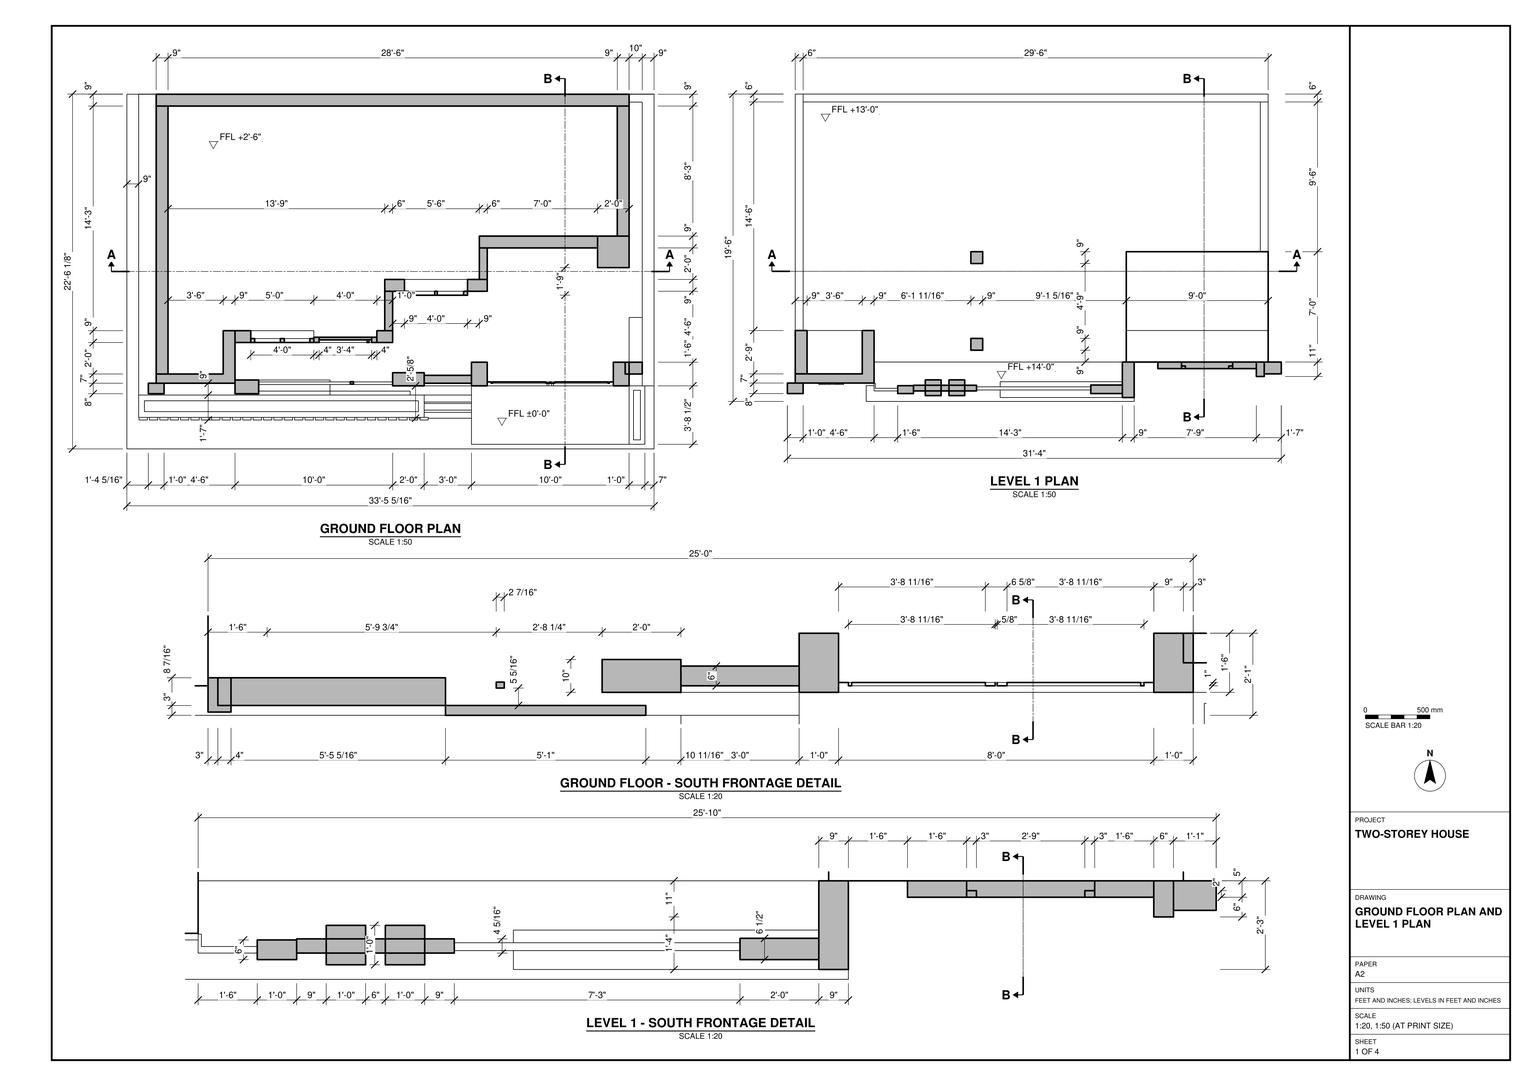
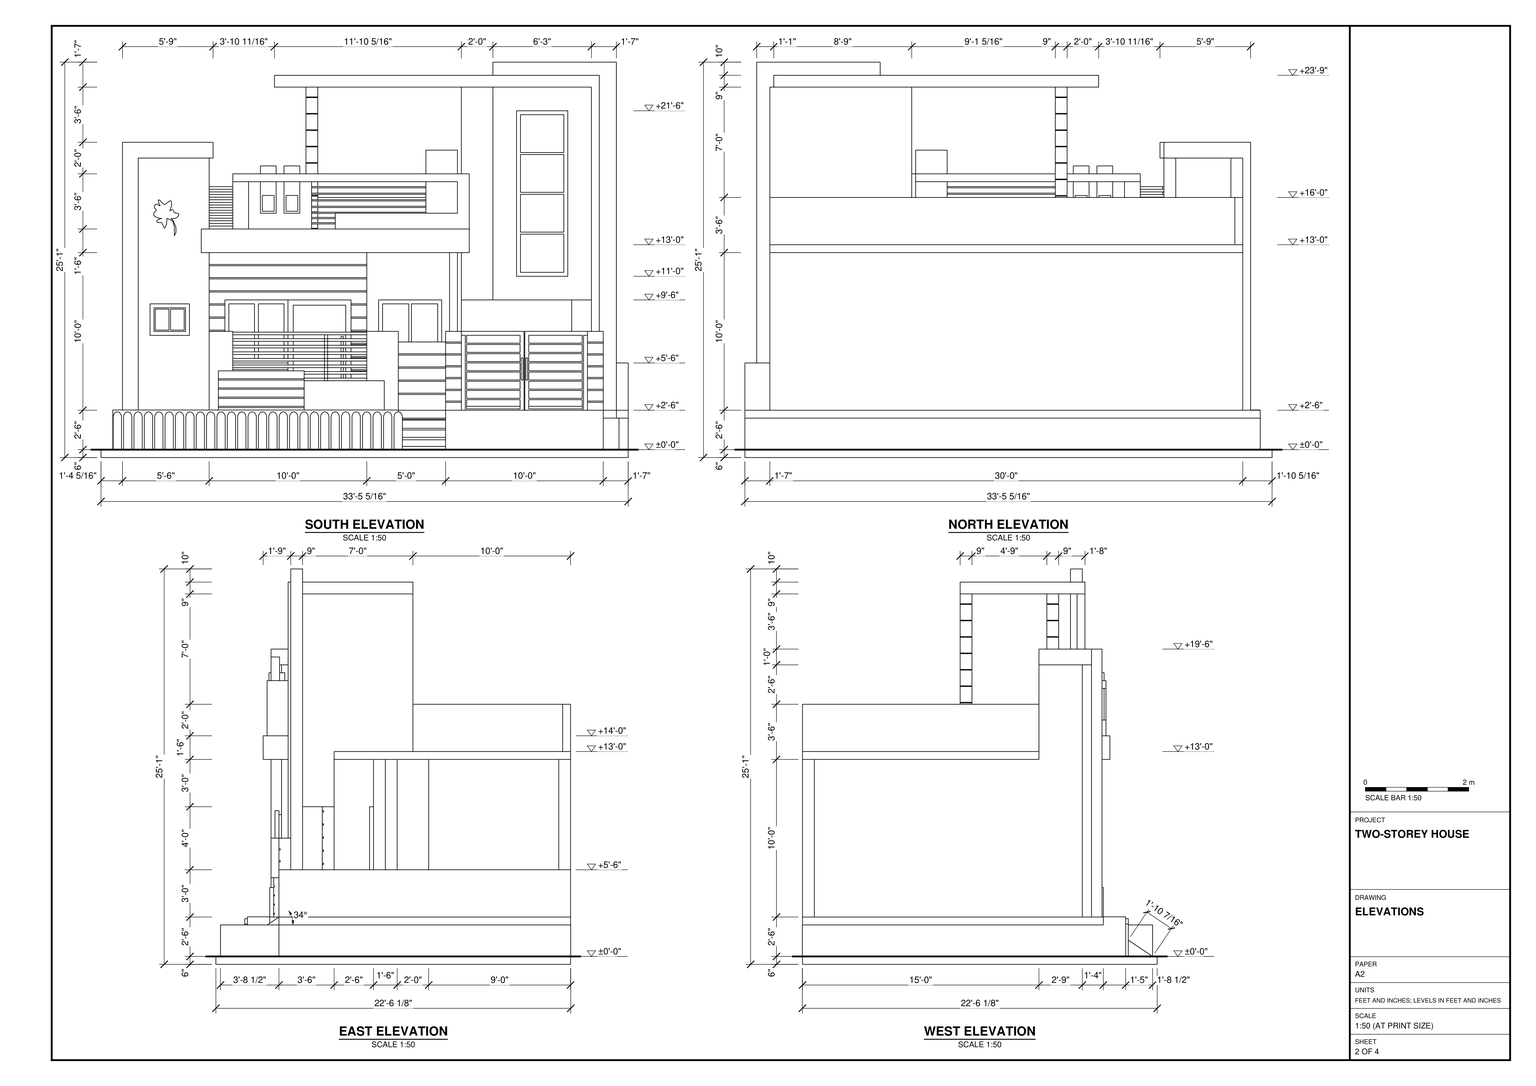
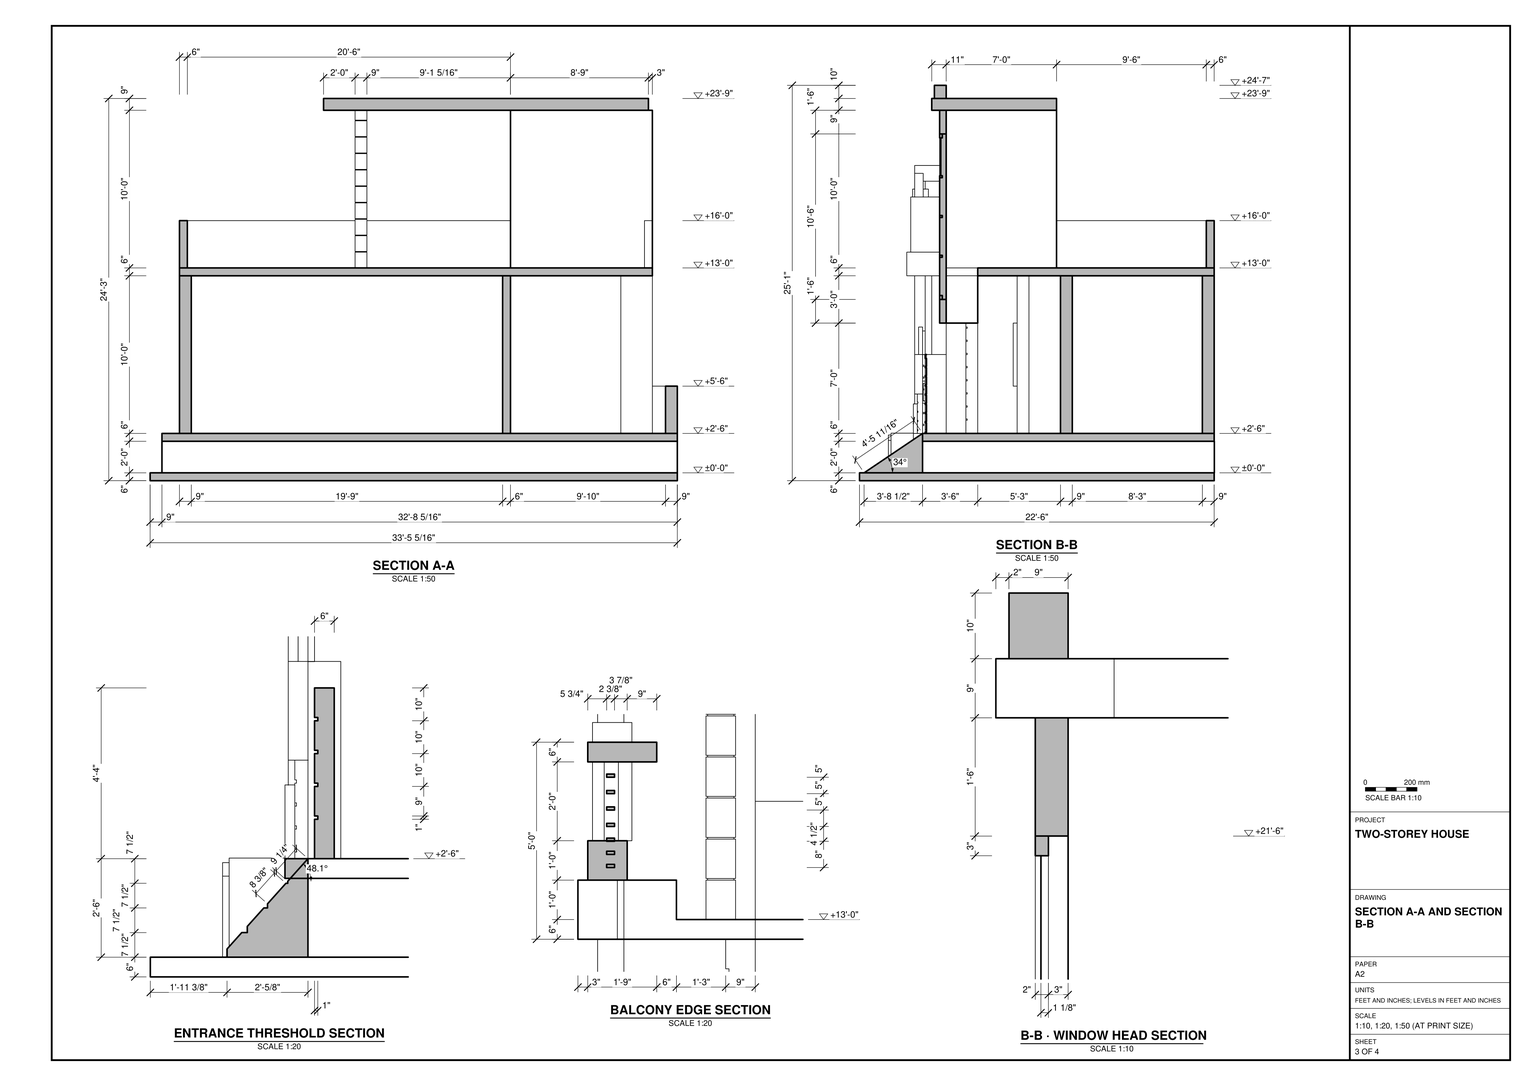
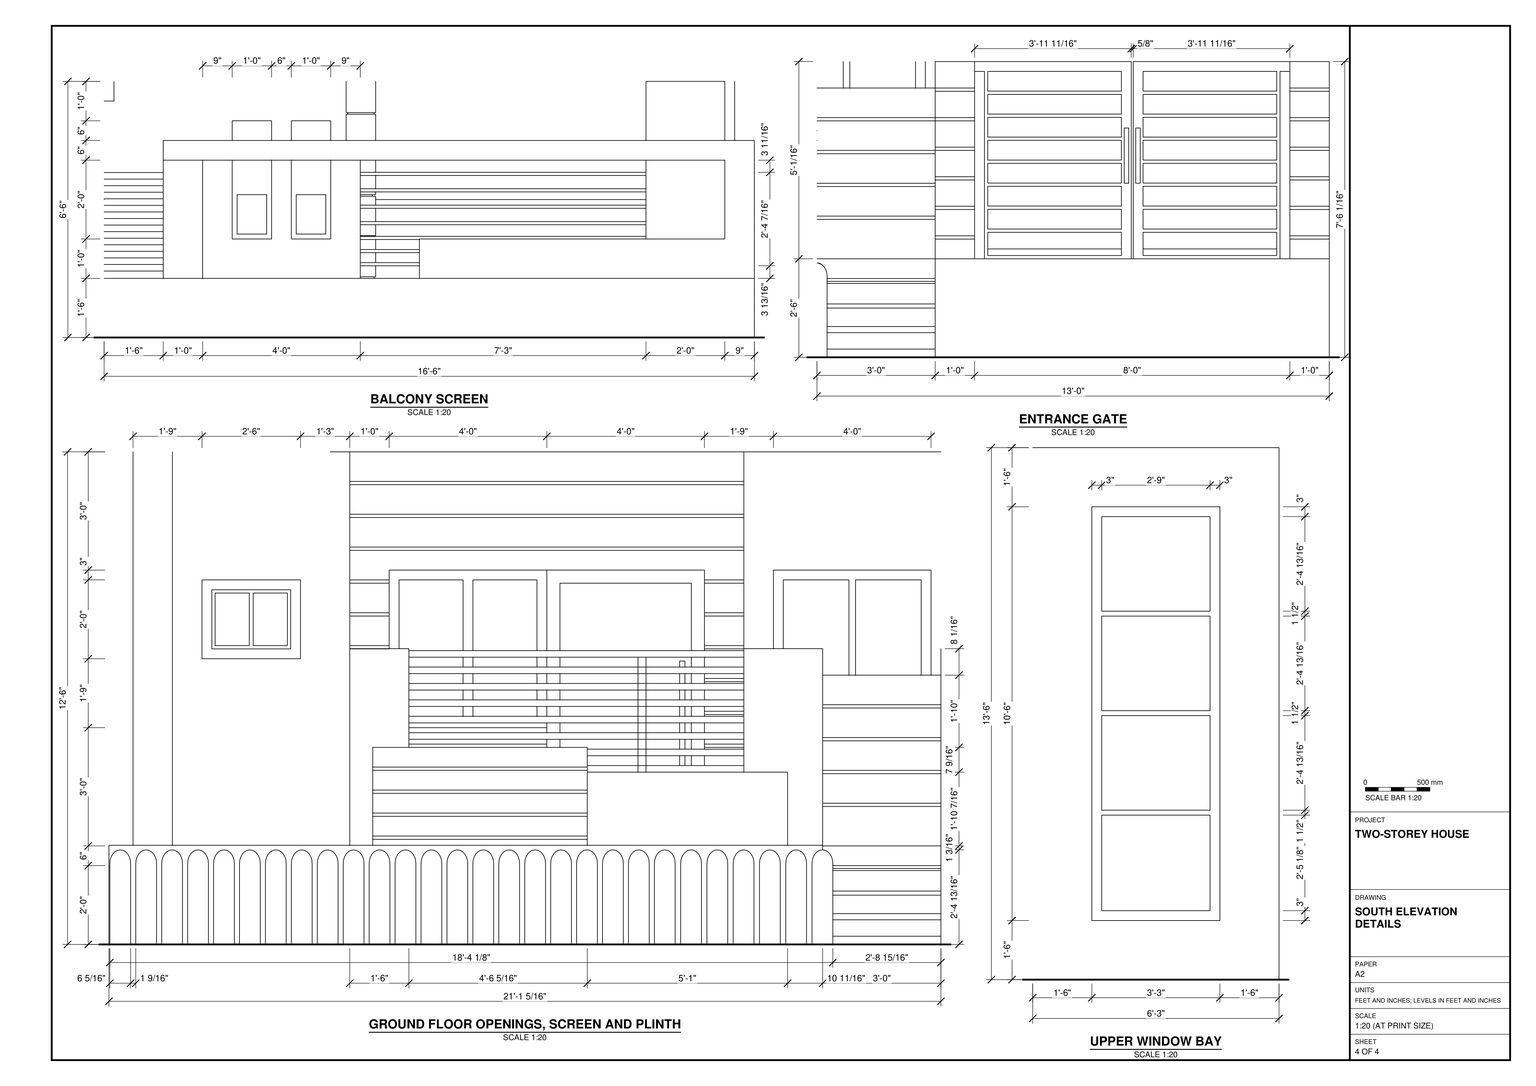
Build the two-storey house in SketchUp using task_files/diagram_01.pdf. Work in feet and inches. The model, including its base, is 33'-5 5/16" wide along X, 22'-6 1/8" deep along Y and 25'-1" high. Use ±0'-0" as the ground datum and +13'-0" as the Level 1 floor level. The raised ground-floor surface is at +2'-6".

Follow the plans for the wall runs, including the stepped outline behind the south frontage. Use the 9" and 6" wall thicknesses where indicated. Use the sections to set the base, plinth, floor slabs, parapets and flat roof canopy. Leave the upper terrace open where the canopy does not cover it.

Build the front approach with the entrance steps and the adjacent ramp leading to the paired gate. Use the enlarged frontage details to position the posts, low walls and horizontal rails. Set the door and window units into the wall openings. On the upper frontage, model the projecting balcony edge, its railing, the canopy supports and the tall window with stacked panes on the right.

Keep walls, slabs and roof elements in separate groups or components. Group each furniture or joinery piece shown separately, and use components for repeated parts. Decor and loose items shown may be any suitable library components. Save one SketchUp model as output_files/two_storey_house_with_a_south_facing_balcony.skp.

# SketchUp Ruby script. Lengths in inches.
U = 1.inch
M = Sketchup.active_model
def pt(a) = Geom::Point3d.new(a.map { |v| v * U })
def face(e, loops, mat)
  f = e.add_face(loops[0].map { |a| pt(a) })
  loops[1..].each { |l| e.add_face(l.map { |a| pt(a) }).erase! }
  f.material = f.back_material = mat if mat
  f
end
# faces: each face lists its corners as indices into pts; further lists are holes
def faces(e, pts, list, mat = nil) = list.each { |f| face(e, (f[0].is_a?(Array) ? f : [f]).map { |l| l.map { |i| pts[i] } }, mat) }
# xy, xz, yz: faces in a plane at the given z, y or x. An outline is a flat list of corners, or four numbers for a rectangle; further outlines are holes
def ring(l) = l.size == 4 ? [[l[0], l[1]], [l[2], l[1]], [l[2], l[3]], [l[0], l[3]]] : l.each_slice(2).to_a
def flat(e, list, mat, &to3) = list.each { |f| face(e, (f[0].is_a?(Array) ? f : [f]).map { |l| ring(l).map { |u, v| to3.(u, v) } }, mat) }
def xy(e, z, list, mat = nil) = flat(e, list, mat) { |x, y| [x, y, z] }
def xz(e, y, list, mat = nil) = flat(e, list, mat) { |x, z| [x, y, z] }
def yz(e, x, list, mat = nil) = flat(e, list, mat) { |y, z| [x, y, z] }
def lines(e, pts, list) = list.each { |a, b| e.add_line(pt(pts[a]), pt(pts[b])) }
# prism: a flat outline (further loops are holes) pulled along v
def prism(e, loops, v, mat = nil)
  f = face(e, loops, mat); d = Geom::Vector3d.new(v.map { |x| x * U })
  f.pushpull(f.normal.samedirection?(d) ? d.length : -d.length)
end
def box(e, o, s, mat = nil) = prism(e, [[o, [o[0] + s[0], o[1], o[2]], [o[0] + s[0], o[1] + s[1], o[2]], [o[0], o[1] + s[1], o[2]]]], [0, 0, s[2]], mat)
def at(x, y, z, deg = 0) = Geom::Transformation.translation(pt([x, y, z])) * Geom::Transformation.rotation(ORIGIN, Z_AXIS, deg.degrees)
def axes(o, x, y, z) = Geom::Transformation.new([*x, 0, *y, 0, *z, 0, *pt(o).to_a, 1])
def part(name) = M.definitions.add(name)
# library, detail: a bought-in or finely detailed component or shape, given as its bounding box
def library(name, o, s) = part(name).tap { |d| box(d.entities, o, s) }
def detail(e, o, s) = box(e.add_group.entities, o, s)
def put(e, d, t, mat = nil) = e.add_instance(d, t).tap { |i| i.material = mat if mat }
def group(e, t, mat = nil) = e.add_group.tap { |g| g.transformation = t; g.material = mat if mat }.entities
root = M.entities
M.materials.add("[Cladding Stucco White]").color = [200, 200, 200]
M.materials.add("[Color D01]").color = [255, 242, 204]
M.materials.add("[Color D02]").color = [255, 229, 153]
M.materials.add("[Color D05]").color = [255, 191, 0]
M.materials.add("[Color E01]").color = [255, 255, 204]
M.materials.add("[Color E03]").color = [122, 122, 48]
M.materials.add("[Color M00]").color = [255, 255, 255]
M.materials.add("[Color M05]").color = [114, 114, 114]
M.materials.add("[Color M06]").color = [86, 86, 86]
M.materials.add("[Color M07]").color = [58, 58, 58]
M.materials.add("[Color M09]").color = [0, 0, 0]
M.materials.add("[Concrete Aggregate Smoke]").color = [154, 150, 148]
M.materials.add("[Grass Dark Green]").color = [106, 157, 55]
M.materials.add("[Metal Aluminum Anodized]").color = [202, 209, 219]
M.materials.add("[Stone Flagstone Ashlar]").color = [221, 147, 129]
M.materials.add("[Stone Sandstone Ashlar Light]").color = [206, 178, 128]
M.materials.add("[Translucent Glass Blue]").color = [100, 149, 237]
M.materials["[Translucent Glass Blue]"].alpha = 0.5
M.materials.add("[Translucent Glass Gray]").color = [128, 128, 128]
M.materials["[Translucent Glass Gray]"].alpha = 0.5
M.materials.add("[Wood Cherry Original]").color = [152, 86, 42]
c1 = part("Group\#32")
prism(c1.entities,[[[18,2,0],[18,0,0],[0,0,0],[0,5.75,0],[1,5.75,0],[1,2,0]]],[0,0,2])
c2 = part("Group\#43")
box(c2.entities,[-12,0,1.4375],[87,2.4,0.96])
c3 = part("Group\#45")
prism(c3.entities,[[[0,0,36],[0,0,0],[12,0,0],[12,0,36]],[[10.5,0,1.5],[1.5,0,1.5],[1.5,0,13.5],[10.5,0,13.5]]],[0,12,0])
c4 = part("Group\#56")
prism(c4.entities,[[[0,2,16.8125],[0,2,15.18],[0,0.63,15.18],[0,0.63,1.63],[0,2,1.63],[0,2,0],[0,0,0],[0,0,16.8125]]],[1.375,0,0])
c5 = part("Group\#61")
box(c5.entities,[0,0,0],[108,2,2])
c6 = part("Group\#67")
prism(c6.entities,[[[0,0,24],[0,0,0],[8.02,0,0],[8.02,0,24],[7.88,0,25.04],[7.48,0,26],[6.84,0,26.83],[6.01,0,27.47],[5.05,0,27.87],[4.01,0,28.01],[2.97,0,27.87],[2,0,27.47],[1.17,0,26.83],[0.54,0,26],[0.14,0,25.04]]],[0,2,0])
c7 = part("Group\#70")
xy(c7.entities,0,[[0,0,9,9]])
xy(c7.entities,12,[[0,0,9,0.5],[0,0.5,0.5,9],[0.5,0.5,8.5,8.5],[8.5,0.5,9,8.5],[0.5,8.5,9,9]])
xy(c7.entities,12.5,[[0,0,9,0.5],[0,0.5,0.5,9],[0.5,0.5,8.5,8.5],[8.5,0.5,9,8.5],[0.5,8.5,9,9]])
xy(c7.entities,24.5,[[0,0,9,0.5],[0,0.5,0.5,9],[0.5,0.5,8.5,8.5],[8.5,0.5,9,8.5],[0.5,8.5,9,9]])
xy(c7.entities,25,[[0,0,9,0.5],[0,0.5,0.5,9],[0.5,0.5,8.5,8.5],[8.5,0.5,9,8.5],[0.5,8.5,9,9]])
xy(c7.entities,37,[[0,0,9,0.5],[0,0.5,0.5,9],[0.5,0.5,8,8.5],[8,0.5,9,8.5],[0.5,8.5,9,9]])
xy(c7.entities,37.5,[[0,0,9,0.5],[0,0.5,0.5,9],[0.5,0.5,8,8.5],[8,0.5,9,8.5],[0.5,8.5,9,9]])
xy(c7.entities,49.5,[[0,0,9,0.5],[0,0.5,0.5,9],[0.5,0.5,8.5,8.5],[8.5,0.5,9,8.5],[0.5,8.5,9,9]])
xy(c7.entities,50,[[0,0,9,0.5],[0,0.5,0.5,9],[0.5,0.5,8.5,8.5],[8.5,0.5,9,8.5],[0.5,8.5,9,9]])
xy(c7.entities,62,[[0,0,9,0.5],[0,0.5,0.5,9],[0.5,0.5,8.5,8.5],[8.5,0.5,9,8.5],[0.5,8.5,9,9]])
xy(c7.entities,62.5,[[0,0,9,0.5],[0,0.5,0.5,9],[0.5,0.5,8.5,8.5],[8.5,0.5,9,8.5],[0.5,8.5,9,9]])
xy(c7.entities,74.5,[[0,0,9,0.5],[0,0.5,0.5,9],[0.5,0.5,8.5,8.5],[8.5,0.5,9,8.5],[0.5,8.5,9,9]])
xy(c7.entities,75,[[0,0,9,0.5],[0,0.5,0.5,9],[0.5,0.5,8.5,8.5],[8.5,0.5,9,8.5],[0.5,8.5,9,9]])
xy(c7.entities,87,[[0,0,9,0.5],[0,0.5,0.5,9],[0.5,0.5,8.5,8.5],[8.5,0.5,9,8.5],[0.5,8.5,9,9]])
xy(c7.entities,87.5,[[0,0,9,0.5],[0,0.5,0.5,9],[0.5,0.5,8.5,8.5],[8.5,0.5,9,8.5],[0.5,8.5,9,9]])
xy(c7.entities,99.5,[[0,0,9,0.5],[0,0.5,0.5,9],[0.5,0.5,8.5,8.5],[8.5,0.5,9,8.5],[0.5,8.5,9,9]])
xy(c7.entities,100,[[0,0,9,0.5],[0,0.5,0.5,9],[0.5,0.5,8.5,8.5],[8.5,0.5,9,8.5],[0.5,8.5,9,9]])
xy(c7.entities,112,[[0,0,9,0.5],[0,0.5,0.5,9],[0.5,0.5,8.5,8.5],[8.5,0.5,9,8.5],[0.5,8.5,9,9]])
xy(c7.entities,112.5,[[0,0,9,0.5],[0,0.5,0.5,9],[0.5,0.5,8.5,8.5],[8.5,0.5,9,8.5],[0.5,8.5,9,9]])
xy(c7.entities,120,[[0,0,9,9]])
xz(c7.entities,0,[[0,0,9,12],[0,12.5,9,24.5],[0,25,9,37],[0,37.5,9,49.5],[0,50,9,62],
  [0,62.5,9,74.5],[0,75,9,87],[0,87.5,9,99.5],[0,100,9,112],[0,112.5,9,120]])
xz(c7.entities,0.5,[[0.5,12,8.5,12.5],[0.5,24.5,8.5,25],[0.5,37,8,37.5],[0.5,49.5,8.5,50],[0.5,62,8.5,62.5],
  [0.5,74.5,8.5,75],[0.5,87,8.5,87.5],[0.5,99.5,8.5,100],[0.5,112,8.5,112.5]])
xz(c7.entities,8.5,[[0.5,12,8.5,12.5],[0.5,24.5,8.5,25],[0.5,37,8,37.5],[0.5,49.5,8.5,50],[0.5,62,8.5,62.5],
  [0.5,74.5,8.5,75],[0.5,87,8.5,87.5],[0.5,99.5,8.5,100],[0.5,112,8.5,112.5]])
xz(c7.entities,9,[[0,0,9,12],[0,12.5,9,24.5],[0,25,9,37],[0,37.5,9,49.5],[0,50,9,62],
  [0,62.5,9,74.5],[0,75,9,87],[0,87.5,9,99.5],[0,100,9,112],[0,112.5,9,120]])
yz(c7.entities,0,[[0,0,9,12],[0,12.5,9,24.5],[0,25,9,37],[0,37.5,9,49.5],[0,50,9,62],
  [0,62.5,9,74.5],[0,75,9,87],[0,87.5,9,99.5],[0,100,9,112],[0,112.5,9,120]])
yz(c7.entities,0.5,[[0.5,12,8.5,12.5],[0.5,24.5,8.5,25],[0.5,37,8.5,37.5],[0.5,49.5,8.5,50],[0.5,62,8.5,62.5],
  [0.5,74.5,8.5,75],[0.5,87,8.5,87.5],[0.5,99.5,8.5,100],[0.5,112,8.5,112.5]])
yz(c7.entities,8,[[0.5,37,8.5,37.5]])
yz(c7.entities,8.5,[[0.5,12,8.5,12.5],[0.5,24.5,8.5,25],[0.5,49.5,8.5,50],[0.5,62,8.5,62.5],[0.5,74.5,8.5,75],
  [0.5,87,8.5,87.5],[0.5,99.5,8.5,100],[0.5,112,8.5,112.5]])
yz(c7.entities,9,[[0,0,9,12],[0,12.5,9,24.5],[0,25,9,37],[0,37.5,9,49.5],[0,50,9,62],
  [0,62.5,9,74.5],[0,75,9,87],[0,87.5,9,99.5],[0,100,9,112],[0,112.5,9,120]])
xy(root,210,[[121.33,40.4375,133.33,52.4375],[139.33,40.4375,151.33,52.4375]])
p = [[247.33,45.5,204],[271.33,45.5,204],[247.33,45.5,210],[271.33,45.5,210],[247.33,48.5,210],[271.33,48.5,210],
  [271.33,42,210],[247.33,42,210],[122.83,44,181.5],[131.83,44,181.5],[131.83,44,193.5],[122.83,44,193.5],
  [121.33,44,180],[133.33,44,180],[133.33,44,204],[133.33,40.4375,204],[121.33,40.4375,204],[121.33,44,204],
  [140.83,44,193.5],[149.83,44,193.5],[149.83,44,181.5],[140.83,44,181.5],[139.33,40.4375,204],[151.33,40.4375,204],
  [151.33,44,204],[151.33,44,180],[139.33,44,180],[139.33,44,204],[160.33,44,204],[160.33,48.32,204],
  [112.33,44,204],[271.33,42,204],[247.33,42,204],[247.33,48.5,204],[271.33,48.5,204],[151.33,52.4375,204],
  [151.33,48.32,204],[151.33,48.32,180],[140.83,48.32,193.5],[149.83,48.32,193.5],[149.83,48.32,181.5],[140.83,48.32,181.5],
  [131.82,48.32,193.5],[122.83,48.32,193.5],[122.83,48.32,181.5],[131.82,48.32,181.5]]
lines(root,p,[[0,1],[2,3],[4,2],[5,4],[6,7],[7,2],[8,9],[9,10],[10,11],[11,8],[12,13],[13,14],
  [14,15],[15,16],[16,17],[17,12],[18,19],[19,20],[20,21],[21,18],[22,23],[23,24],[24,25],[25,26],
  [26,27],[27,22],[28,29],[24,28],[17,30],[27,14],[31,32],[32,0],[0,33],[33,34],[35,36],[36,37],
  [38,39],[39,40],[40,41],[41,38],[42,43],[43,44],[44,45],[45,42]])
g1 = group(root,at(82.33,81,30),"[Color D01]")
xy(g1,0,[[0,0,60,9],[108,0,120,9]])
xy(g1,10,[[0,0,60,1],[108,0,120,1]])
xy(g1,11,[[0,0,60,1],[108,0,120,1]])
xy(g1,20,[[0,0,60,1],[108,0,120,1]])
xy(g1,21,[[0,0,60,1],[108,0,120,1]])
xy(g1,30,[[0,0,60,1],[108,0,120,1]])
xy(g1,31,[[0,0,60,1],[108,0,120,1]])
xy(g1,36,[[12,0,60,9]])
xy(g1,40,[[0,0,12,1],[108,0,120,1]])
xy(g1,41,[[0,0,12,1],[108,0,120,1]])
xy(g1,50,[[0,0,12,1],[108,0,120,1]])
xy(g1,51,[[0,0,12,1],[108,0,120,1]])
xy(g1,60,[[0,0,12,1],[108,0,120,1]])
xy(g1,61,[[0,0,12,1],[108,0,120,1]])
xy(g1,70,[[0,0,12,1],[108,0,120,1]])
xy(g1,71,[[0,0,12,1],[108,0,120,1]])
xy(g1,80,[[0,0,12,1],[108,0,120,1]])
xy(g1,81,[[0,0,12,1],[108,0,120,1]])
xy(g1,84,[[12,0,60,9],[60,0,108,9]])
xy(g1,90,[[0,0,120,1]])
xy(g1,91,[[0,0,120,1]])
xy(g1,100,[[0,0,120,1]])
xy(g1,101,[[0,0,120,1]])
xy(g1,110,[[0,0,120,1]])
xy(g1,111,[[0,0,120,1]])
xy(g1,120,[[0,0,120,9]])
xz(g1,0,[[0,0,60,10],[108,0,120,10],[0,11,60,20],[108,11,120,20],[0,21,60,30],
  [108,21,120,30],[0,31,60,31,60,36,12,36,12,40,0,40],[108,31,120,40],[0,41,12,50],[108,41,120,50],
  [0,51,12,60],[108,51,120,60],[0,61,12,70],[108,61,120,70],[0,71,12,80],
  [108,71,120,80],[0,81,12,81,12,84,108,84,108,81,120,81,120,90,0,90],[0,91,120,100],[0,101,120,110],[0,111,120,120]])
xz(g1,1,[[0,10,60,11],[108,10,120,11],[0,20,60,21],[108,20,120,21],[0,30,60,31],
  [108,30,120,31],[0,40,12,41],[108,40,120,41],[0,50,12,51],[108,50,120,51],
  [0,60,12,61],[108,60,120,61],[0,70,12,71],[108,70,120,71],[0,80,12,81],
  [108,80,120,81],[0,90,120,91],[0,100,120,101],[0,110,120,111]])
xz(g1,9,[[0,0,0,120,120,120,120,0,108,0,108,84,12,84,12,36,60,36,60,0]])
yz(g1,0,[[0,0,0,10,1,10,1,11,0,11,0,20,1,20,1,21,0,21,0,30,1,30,1,31,0,31,0,40,1,40,1,41,0,41,0,50,1,50,1,51,0,51,0,60,1,60,1,61,0,61,0,70,1,70,1,71,0,71,0,80,1,80,1,81,0,81,0,90,1,90,1,91,0,91,0,100,1,100,1,101,0,101,0,110,1,110,1,111,0,111,0,120,9,120,9,0]])
yz(g1,12,[[0,36,9,36,9,84,0,84,0,81,1,81,1,80,0,80,0,71,1,71,1,70,0,70,0,61,1,61,1,60,0,60,0,51,1,51,1,50,0,50,0,41,1,41,1,40,0,40]])
yz(g1,60,[[0,0,9,0,9,36,0,36,0,31,1,31,1,30,0,30,0,21,1,21,1,20,0,20,0,11,1,11,1,10,0,10]])
yz(g1,108,[[0,0,0,10,1,10,1,11,0,11,0,20,1,20,1,21,0,21,0,30,1,30,1,31,0,31,0,40,1,40,1,41,0,41,0,50,1,50,1,51,0,51,0,60,1,60,1,61,0,61,0,70,1,70,1,71,0,71,0,80,1,80,1,81,0,81,0,84,9,84,9,0]])
yz(g1,120,[[0,0,9,0,9,120,0,120,0,111,1,111,1,110,0,110,0,101,1,101,1,100,0,100,0,91,1,91,1,90,0,90,0,81,1,81,1,80,0,80,0,71,1,71,1,70,0,70,0,61,1,61,1,60,0,60,0,51,1,51,1,50,0,50,0,41,1,41,1,40,0,40,0,31,1,31,1,30,0,30,0,21,1,21,1,20,0,20,0,11,1,11,1,10,0,10]])
g2 = group(root,at(94.33,81,66),"[Color M09]")
prism(g2,[[[0,0,0],[48,0,0],[48,0,48],[0,0,48]],[[22.5,0,45],[22.5,0,3],[3,0,3],[3,0,45]],[[25.5,0,45],[45,0,45],[45,0,3],[25.5,0,3]]],[0,3,0])
g3 = group(root,at(142.33,81,30),"[Wood Cherry Original]")
prism(g3,[[[0,4,0],[0,4,84],[48,4,84],[48,4,0]],[[4,4,80],[4,4,4],[44,4,4],[44,4,80]]],[0,-4,0])
g4 = group(root,at(146.33,83,34),"[Wood Cherry Original]")
box(g4,[0,0,0],[40,2,76])
g5 = group(root,at(182.78,81,49.66),"[Metal Aluminum Anodized]")
prism(g5,[[[1.625,2,35],[1.625,2,36.625],[1.625,0,36.625],[1.625,0,0],[1.625,2,0],[1.625,2,1.625],[1.625,0.625,1.625],[1.625,0.625,35]]],[-1.625,0,0])
g6 = group(root,at(196.33,120,30),"[Color D05]")
prism(g6,[[[78,9,0],[0,9,0],[0,9,120],[78,9,120]],[[15,9,84],[15,9,36],[63,9,36],[63,9,84]]],[0,-9,0])
g7 = group(root,at(196.33,90,30))
box(g7,[0,0,0],[6,30,120])
g8 = group(root,at(211.33,117,66),"[Color M09]")
prism(g8,[[[0,3,48],[48,3,48],[48,3,0],[0,3,0]],[[23,3,3],[23,3,45],[3,3,45],[3,3,3]],[[45,3,45],[25,3,45],[25,3,3],[45,3,3]]],[0,-3,0])
g9 = group(root,at(268.33,153,30),"[Color E03]")
box(g9,[0,0,0],[90,9,120])
g10 = group(root,at(268.33,129,30))
box(g10,[0,0,0],[6,24,120])
g11 = group(root,at(358.33,138,30),"[Color E03]")
box(g11,[0,0,0],[24,24,120],"[Color D05]")
g12 = group(root,at(22.33,48,30),"[Color D05]")
xy(g12,0,[[0,2,0,9,51,9,51,42,60,42,60,2]])
xy(g12,60,[[18,2,42,9]])
xy(g12,78,[[18,2,42,9]])
xy(g12,192,[[0,2,60,2,60,42,51,42,51,9,0,9]])
xz(g12,2,[[[0,0,60,192],[18,60,42,78]]])
xz(g12,9,[[[0,0,51,192],[18,60,42,78]]])
xz(g12,42,[[51,0,60,192]])
yz(g12,0,[[2,0,9,192]])
yz(g12,18,[[2,60,9,78]])
yz(g12,42,[[2,60,9,78]])
yz(g12,51,[[9,0,42,192]])
yz(g12,60,[[2,0,42,192]])
g13 = group(root,at(22.33,57,30))
prism(g13,[[[0,204,0],[0,0,0],[0,0,192],[0,33,192],[0,33,120],[0,204,120]]],[9,0,0])
g14 = group(root,at(373.33,162,30))
box(g14,[0,0,0],[9,99,120])
g15 = group(root,at(22.33,90,150),"[Color M00]")
xy(g15,0,[[54,-54,54,-42,60,-42,60,0,0,0,0,180,360,180,360,0,252,0,252,-24,258,-24,258,-54]])
xy(g15,6,[[60,-24,252,-24,252,0,360,0,360,180,0,180,0,0,60,0]])
xy(g15,18,[[54,-54,258,-54,258,-24,60,-24,60,-42,54,-42]])
xz(g15,-54,[[54,0,258,18]])
xz(g15,-42,[[54,0,60,18]])
xz(g15,-24,[[252,0,258,6],[60,6,258,18]])
xz(g15,0,[[0,0,60,6],[252,0,360,6]])
xz(g15,180,[[0,0,360,6]])
yz(g15,0,[[0,0,180,6]])
yz(g15,54,[[-54,0,-42,18]])
yz(g15,60,[[-42,0,-42,18,-24,18,-24,6,0,6,0,0]])
yz(g15,252,[[-24,0,0,6]])
yz(g15,258,[[-54,0,-24,18]])
yz(g15,360,[[0,0,180,6]])
g16 = group(root,at(262.33,48,30),"[Color M07]")
prism(g16,[[[12,0,0],[12,18,0],[12,18,60.0625],[12,0,60.0625],[12,0,52],[12,1,52],[12,1,51],[12,0,51],[12,0,43],[12,1,43],[12,1,42],[12,0,42],[12,0,34],[12,1,34],[12,1,33],[12,0,33],[12,0,25],[12,1,25],[12,1,24],[12,0,24],[12,0,16],[12,1,16],[12,1,15],[12,0,15],[12,0,7],[12,1,7],[12,1,6],[12,0,6]]],[-12,0,0])
g17 = group(root,at(274.33,66,114),"[Color M06]")
prism(g17,[[[108,24,0],[108,24,42],[108,84,42],[108,84,162],[108,0,162],[108,0,0]]],[-108,0,0])
g18 = group(root,at(370.33,48,30),"[Color M07]")
prism(g18,[[[12,0,0],[12,18,0],[12,18,60.0625],[12,0,60.0625],[12,0,52],[12,1,52],[12,1,51],[12,0,51],[12,0,43],[12,1,43],[12,1,42],[12,0,42],[12,0,34],[12,1,34],[12,1,33],[12,0,33],[12,0,25],[12,1,25],[12,1,24],[12,0,24],[12,0,16],[12,1,16],[12,1,15],[12,0,15],[12,0,7],[12,1,7],[12,1,6],[12,0,6]]],[-12,0,0])
g19 = group(root,at(373.33,51,150.0625))
xy(g19,-60,[[0,4,6,15]])
xy(g19,125.9375,[[[-241.3125,4,0,99],[-195,22,-183,81],[-177,22,-165,81],[-159,22,-147,81],[-141,22,-129,81],[-123,22,-111,81]],[0,15,6,99]])
xy(g19,134.9375,[[[-241.3125,4,6,99],[-195,22,-183,81],[-177,22,-165,81],[-159,22,-147,81],[-141,22,-129,81],[-123,22,-111,81]]])
xz(g19,4,[[0,-60,6,-60,6,134.9375,-241.3125,134.9375,-241.3125,125.9375,0,125.9375]])
xz(g19,15,[[0,-60,6,125.9375]])
xz(g19,22,[[-195,125.9375,-183,134.9375],[-177,125.9375,-165,134.9375],[-159,125.9375,-147,134.9375],[-141,125.9375,-129,134.9375],[-123,125.9375,-111,134.9375]])
xz(g19,81,[[-195,125.9375,-183,134.9375],[-177,125.9375,-165,134.9375],[-159,125.9375,-147,134.9375],[-141,125.9375,-129,134.9375],[-123,125.9375,-111,134.9375]])
xz(g19,99,[[-241.3125,125.9375,6,134.9375]])
yz(g19,-241.3125,[[4,125.9375,99,134.9375]])
yz(g19,-195,[[22,125.9375,81,134.9375]])
yz(g19,-183,[[22,125.9375,81,134.9375]])
yz(g19,-177,[[22,125.9375,81,134.9375]])
yz(g19,-165,[[22,125.9375,81,134.9375]])
yz(g19,-159,[[22,125.9375,81,134.9375]])
yz(g19,-147,[[22,125.9375,81,134.9375]])
yz(g19,-141,[[22,125.9375,81,134.9375]])
yz(g19,-129,[[22,125.9375,81,134.9375]])
yz(g19,-123,[[22,125.9375,81,134.9375]])
yz(g19,-111,[[22,125.9375,81,134.9375]])
yz(g19,0,[[4,-60,15,125.9375]])
yz(g19,6,[[4,-60,15,-60,15,125.9375,99,125.9375,99,134.9375,4,134.9375]])
g20 = group(root,at(298.33,61,114),"[Concrete Aggregate Smoke]")
prism(g20,[[[75,5,162],[75,5,0],[0,5,0],[0,5,162]],[[57,5,18],[57,5,144],[18,5,144],[18,5,18]]],[0,-5,0])
g21 = group(root,at(316.33,61,132),"[Color M09]")
prism(g21,[[[0,2,126],[39,2,126],[39,2,0],[0,2,0]],[[36,2,32.1],[3,2,32.1],[3,2,3],[36,2,3]],[[3,2,62.4],[3,2,33.6],[36,2,33.6],[36,2,62.4]],[[3,2,63.9],[36,2,63.9],[36,2,92.7],[3,2,92.7]],[[3,2,123],[3,2,94.2],[36,2,94.2],[36,2,123]]],[0,-2,0])
g22 = group(root,at(319.33,61,135),"[Translucent Glass Blue]")
xz(g22,0,[[0,0,33,29.1]])
g23 = group(root,at(319.33,61,165.6),"[Translucent Glass Blue]")
xz(g23,0,[[0,0,33,28.8]])
g24 = group(root,at(319.33,61,226.2),"[Translucent Glass Blue]")
p = [[33,2,0],[0,0,0],[0,0,28.8],[33,2,28.8]]
faces(g24,p,[[0,1,2,3]])
g25 = group(root,at(319.33,61,195.9),"[Translucent Glass Blue]")
xz(g25,0,[[0,0,33,28.8]])
g26 = group(root,at(265.33,55,90.0625))
box(g26,[0,0,0],[6,11,59.9375])
g27 = group(root,at(172.33,42,168),"[Color D05]")
xy(g27,0,[[6,-3,6,9,99,9,99,24,108,24,108,-3]])
xy(g27,12,[[6,-3,99,9]])
xy(g27,36,[[-72,-3,99,18]])
xy(g27,42,[[-72,-3,108,-3,108,24,99,24,99,18,-72,18]])
xz(g27,-3,[[6,0,108,0,108,42,-72,42,-72,36,99,36,99,12,6,12]])
xz(g27,9,[[6,0,99,12]])
xz(g27,18,[[-72,36,99,42]])
xz(g27,24,[[99,0,108,42]])
yz(g27,-72,[[-3,36,18,42]])
yz(g27,6,[[-3,0,9,12]])
yz(g27,99,[[9,0,9,12,-3,12,-3,36,18,36,18,42,24,42,24,0]])
yz(g27,108,[[-3,0,24,42]])
g28 = group(root,at(247.33,45.5,180),"[Color M06]")
box(g28,[0,-3.5,0],[24,6.5,48])
g29 = group(root,at(100.33,39,168),"[Color D05]")
box(g29,[0,3,0],[12,6,36])
g30 = group(root,at(82.33,44,170.24),"[Color M05]")
put(g30,c1,at(0,0,20))
put(g30,c1,at(0,0,16))
put(g30,c1,at(0,0,28))
put(g30,c1,at(0,0,0))
put(g30,c1,at(0,0,24))
put(g30,c1,at(0,0,12))
put(g30,c1,at(0,0,4))
put(g30,c1,at(0,0,8))
g31 = group(root,at(124.33,44.32,172.61),"[Color M06]")
box(g31,[-12,-0.32,-4.61],[48,4.32,40.61])
g32 = group(root,at(160.33,44.75,181.84),"[Color M05]")
g33 = group(g32,at(12,0,11.0625))
box(g33,[-12,0,1.4375],[87,2.4,0.96])
g34 = group(g32,at(12,0,1.0625))
box(g34,[-12,0,1.4375],[87,2.4,0.96])
g35 = group(g32,at(12,0,16.0625))
box(g35,[-12,0,1.4375],[87,2.4,0.96])
g36 = group(g32,at(12,0,6.0625))
box(g36,[-12,0,1.4375],[87,2.4,0.96])
put(g32,c2,at(12,0,-3.4375))
put(g32,c2,at(12,0,-7.4375))
put(g32,c2,at(12,0,-11.4375))
put(root,c3,at(121.33,40.4375,180))
put(root,c3,at(139.33,40.4375,180))
g37 = group(root,at(22.33,90,156))
box(g37,[0,0,0],[6,180,36])
g38 = group(root,at(28.33,264,156))
box(g38,[0,0,0],[354,6,36])
g39 = group(root,at(376.33,150,156))
box(g39,[0,0,0],[6,114,36])
g40 = group(root,at(40.33,57,90))
xz(g40,0,[[0,0,24,18]])
g41 = group(root,at(37.33,45,87))
prism(g41,[[[0,0,24],[0,0,0],[30,0,0],[30,0,24]],[[3,0,21],[27,0,21],[27,0,3],[3,0,3]]],[0,3,0])
g42 = group(root,at(40.33,48,90),"[Color M09]")
prism(g42,[[[0,2,0],[0,2,18],[24,2,18],[24,2,0]],[[11.4,2,1],[11.4,2,17],[1,2,17],[1,2,1]],[[23,2,17],[12.6,2,17],[12.6,2,1],[23,2,1]]],[0,-2,0])
g43 = group(root,at(52.93,48,91),"[Translucent Glass Gray]")
xz(g43,0,[[0,0,10.4,16]])
g44 = group(root,at(41.33,48,91),"[Translucent Glass Gray]")
xz(g44,0,[[0,0,10.4,16]])
g45 = group(root,at(22.33,42,30),"[Concrete Aggregate Smoke]")
xy(g45,0,[[-6,0,6,8]])
xy(g45,192,[[6,0,6,8,60,8,60,48,63,48,63,0]])
xy(g45,204,[[-6,0,63,0,63,48,60,48,60,8,-6,8]])
xz(g45,0,[[-6,0,6,0,6,192,63,192,63,204,-6,204]])
xz(g45,8,[[-6,0,-6,204,60,204,60,192,6,192,6,0]])
xz(g45,48,[[60,192,63,204]])
yz(g45,-6,[[0,0,8,204]])
yz(g45,6,[[0,0,8,192]])
yz(g45,60,[[8,192,48,204]])
yz(g45,63,[[0,192,48,204]])
g46 = group(root,at(274.33,48,30))
xy(g46,0,[[3,2,47.7,3],[48.3,2,93,3]])
xy(g46,1,[[4,2,44.7,3],[51.3,2,92,3]])
xy(g46,8.0625,[[4,2,44.7,3],[51.3,2,92,3]])
xy(g46,9.0625,[[4,2,44.7,3],[51.3,2,92,3]])
xy(g46,15.0625,[[4,2,44.7,3],[51.3,2,92,3]])
xy(g46,16.0625,[[4,2,44.7,3],[51.3,2,92,3]])
xy(g46,22.0625,[[4,2,44.7,3],[51.3,2,92,3]])
xy(g46,23.0625,[[4,2,44.7,3],[51.3,2,92,3]])
xy(g46,29.0625,[[4,2,44.7,3],[51.3,2,92,3]])
xy(g46,30.0625,[[4,2,44.7,3],[51.3,2,92,3]])
xy(g46,36.0625,[[4,2,44.7,3],[51.3,2,92,3]])
xy(g46,37.0625,[[4,2,44.7,3],[51.3,2,92,3]])
xy(g46,43.0625,[[4,2,44.7,3],[51.3,2,92,3]])
xy(g46,44.0625,[[4,2,44.7,3],[51.3,2,92,3]])
xy(g46,50.0625,[[4,2,44.7,3],[51.3,2,92,3]])
xy(g46,51.0625,[[4,2,44.7,3],[51.3,2,92,3]])
xy(g46,57.0625,[[0,2,3,3],[4,2,44.7,3],[51.3,2,92,3],[93,2,96,3]])
xy(g46,60.0625,[[0,2,47.7,3],[48.3,2,96,3]])
xz(g46,2,[[[3,0,3,57.0625,0,57.0625,0,60.0625,47.7,60.0625,47.7,0],[4,1,44.7,8.0625],[4,23.0625,44.7,29.0625],[4,51.0625,44.7,57.0625],[4,44.0625,44.7,50.0625],[4,37.0625,44.7,43.0625],[4,30.0625,44.7,36.0625],[4,9.0625,44.7,15.0625],[4,16.0625,44.7,22.0625]],[[48.3,0,48.3,60.0625,96,60.0625,96,57.0625,93,57.0625,93,0],[51.3,1,92,8.0625],[51.3,9.0625,92,15.0625],[51.3,16.0625,92,22.0625],[51.3,23.0625,92,29.0625],[51.3,30.0625,92,36.0625],[51.3,51.0625,92,57.0625],[51.3,44.0625,92,50.0625],[51.3,37.0625,92,43.0625]]],"[Color M00]")
xz(g46,3,[[4,9.0625,44.7,15.0625],[51.3,9.0625,92,15.0625],[4,16.0625,44.7,22.0625],[51.3,16.0625,92,22.0625],[4,23.0625,44.7,29.0625],
  [51.3,23.0625,92,29.0625],[4,30.0625,44.7,36.0625],[51.3,30.0625,92,36.0625],[4,37.0625,44.7,43.0625],[51.3,37.0625,92,43.0625],
  [4,44.0625,44.7,50.0625],[51.3,44.0625,92,50.0625],[4,51.0625,44.7,57.0625],[51.3,51.0625,92,57.0625]],"[Color D05]")
xz(g46,3,[[0,0,3,57.0625],[93,0,96,57.0625],[4,1,44.7,3],[51.3,1,92,3],[4,3,44.7,8.0625],
  [51.3,3,92,8.0625]],"[Color M09]")
yz(g46,0,[[2,57.0625,3,60.0625]])
yz(g46,3,[[2,0,3,57.0625]])
yz(g46,4,[[2,1,3,3],[2,3,3,8.0625],[2,9.0625,3,15.0625],[2,16.0625,3,22.0625],[2,23.0625,3,29.0625],
  [2,30.0625,3,36.0625],[2,37.0625,3,43.0625],[2,44.0625,3,50.0625],[2,51.0625,3,57.0625]])
yz(g46,44.7,[[2,1,3,3],[2,3,3,8.0625],[2,9.0625,3,15.0625],[2,16.0625,3,22.0625],[2,23.0625,3,29.0625],
  [2,30.0625,3,36.0625],[2,37.0625,3,43.0625],[2,44.0625,3,50.0625],[2,51.0625,3,57.0625]])
yz(g46,47.7,[[2,0,3,60.0625]])
yz(g46,48.3,[[2,0,3,60.0625]])
yz(g46,51.3,[[2,1,3,3],[2,3,3,8.0625],[2,9.0625,3,15.0625],[2,16.0625,3,22.0625],[2,23.0625,3,29.0625],
  [2,30.0625,3,36.0625],[2,37.0625,3,43.0625],[2,44.0625,3,50.0625],[2,51.0625,3,57.0625]])
yz(g46,92,[[2,1,3,3],[2,3,3,8.0625],[2,9.0625,3,15.0625],[2,16.0625,3,22.0625],[2,23.0625,3,29.0625],
  [2,30.0625,3,36.0625],[2,37.0625,3,43.0625],[2,44.0625,3,50.0625],[2,51.0625,3,57.0625]])
yz(g46,93,[[2,0,3,57.0625]])
yz(g46,96,[[2,57.0625,3,60.0625]])
put(root,c4,at(319.89,48,53.01),"[Metal Aluminum Anodized]")
put(root,c4,at(323.39,48,53.01),"[Metal Aluminum Anodized]")
g47 = group(root,at(226.33,50,30),"[Color E01]")
prism(g47,[[[36,0,0],[36,6,0],[36,6,52],[36,0,52],[36,0,43],[36,1,43],[36,1,42],[36,0,42],[36,0,33],[36,1,33],[36,1,32],[36,0,32],[36,0,23],[36,1,23],[36,1,22],[36,0,22],[36,0,13],[36,1,13],[36,1,12],[36,0,12]]],[-36,0,0])
g48 = group(root,at(202.33,48,30),"[Concrete Aggregate Smoke]")
box(g48,[0,0,0],[24,10,60.0625])
g49 = group(root,at(82.33,42,30),"[Concrete Aggregate Smoke]")
prism(g49,[[[0,0,0],[7,0,0],[7,0,30],[18,0,30],[18,0,60.0625],[0,0,60.0625]]],[0,10.4375,0])
g50 = group(root,at(85.33,44,30))
xy(g50,0,[[0,0,69.3125,8.4375]])
xy(g50,2,[[0,0,69.3125,0.5]])
xy(g50,3,[[0,0,69.3125,0.5]])
xy(g50,9,[[0,0,69.3125,0.5]])
xy(g50,10,[[0,0,69.3125,0.5]])
xy(g50,16,[[0,0,69.3125,0.5]])
xy(g50,17,[[0,0,69.3125,0.5]])
xy(g50,23,[[0,0,69.3125,0.5]])
xy(g50,24,[[0,0,69.3125,0.5]])
xy(g50,30,[[0,0,69.3125,8.4375]])
xz(g50,0,[[0,0,69.3125,2],[0,3,69.3125,9],[0,10,69.3125,16],[0,17,69.3125,23],[0,24,69.3125,30]],"[Color M06]")
xz(g50,0.5,[[0,2,69.3125,3],[0,9,69.3125,10],[0,16,69.3125,17],[0,23,69.3125,24]])
xz(g50,8.4375,[[0,0,69.3125,30]])
yz(g50,0,[[0,0,0,2,0.5,2,0.5,3,0,3,0,9,0.5,9,0.5,10,0,10,0,16,0.5,16,0.5,17,0,17,0,23,0.5,23,0.5,24,0,24,0,30,8.4375,30,8.4375,0]])
yz(g50,69.3125,[[0,0,8.4375,0,8.4375,30,0,30,0,24,0.5,24,0.5,23,0,23,0,17,0.5,17,0.5,16,0,16,0,10,0.5,10,0.5,9,0,9,0,3,0.5,3,0.5,2,0,2]])
put(root,c5,at(94.33,49,87.46),"[Color M05]")
put(root,c5,at(94.33,49,82.46),"[Color M05]")
put(root,c5,at(94.33,49,77.46),"[Color M05]")
put(root,c5,at(94.33,49,72.46),"[Color M05]")
put(root,c5,at(94.33,49,67.46),"[Color M05]")
put(root,c5,at(94.33,49,62.46),"[Color M05]")
put(root,c5,at(94.33,49,57.46),"[Color M05]")
put(root,c5,at(94.33,49,52.46),"[Color M05]")
g51 = group(root,at(132.33,41,30),"[Color M00]")
box(g51,[22.32,0,0],[61,3,22.46])
g52 = group(root,at(170.1,49,30),"[Color M05]")
box(g52,[0,0.3,0],[2.4375,1.82,57.46])
g53 = group(root,at(298.33,57,30),"[Concrete Aggregate Smoke]")
xy(g53,-6,[[84,-9,84,0,81,0,81,9,94,9,94,-9]])
xy(g53,0,[[84,-9,94,0]])
xy(g53,255,[[0,0,81,9]])
xy(g53,265,[[0,0,94,9]])
xz(g53,-9,[[84,-6,94,0]])
xz(g53,0,[[81,-6,84,60.0625],[84,0,94,0,94,265,0,265,0,255,81,255,81,60.0625,84,60.0625]])
xz(g53,9,[[81,-6,81,255,0,255,0,265,94,265,94,-6]])
yz(g53,0,[[0,255,9,265]])
yz(g53,81,[[0,-6,9,255]])
yz(g53,84,[[-9,-6,0,0]])
yz(g53,94,[[-9,-6,9,-6,9,265,0,265,0,0,-9,0]])
g54 = group(root,at(9,41,0))
xy(g54,0,[[0,-17,0,229.125,392.33,229.125,392.33,7,217.33,7,217.33,-17]])
xy(g54,24,[[0,0,217.33,0,217.33,7,392.33,7,392.33,229.125,0,229.125]])
xy(g54,28.4375,[[4.375,-12.625,212.96,-4.375]],"[Grass Dark Green]")
xy(g54,30.1875,[[[0,-17,217.33,0],[4.375,-12.625,212.96,-4.375]]],"[Stone Sandstone Ashlar Light]")
xz(g54,-17,[[0,0,217.33,30.1875]],"[Stone Sandstone Ashlar Light]")
xz(g54,-12.625,[[4.375,28.4375,212.96,30.1875]],"[Stone Sandstone Ashlar Light]")
xz(g54,-4.375,[[4.375,28.4375,13.33,30.1875],[13.33,28.4375,212.96,30.1875]],"[Stone Sandstone Ashlar Light]")
xz(g54,0,[[0,24,13.33,30.1875],[13.33,24,217.33,30.1875]])
xz(g54,7,[[217.33,0,373.33,24],[373.33,0,392.33,24]])
xz(g54,229.125,[[0,0,392.33,24]])
yz(g54,0,[[-17,0,-17,30.1875,0,30.1875,0,24,229.125,24,229.125,0]])
yz(g54,4.375,[[-12.625,28.4375,-4.375,30.1875]],"[Stone Sandstone Ashlar Light]")
yz(g54,212.96,[[-12.625,28.4375,-4.375,30.1875]],"[Stone Sandstone Ashlar Light]")
yz(g54,217.33,[[-17,0,7,0,7,24,0,24,0,30.1875,-17,30.1875]],"[Stone Sandstone Ashlar Light]")
yz(g54,392.33,[[7,0,229.125,24]])
g55 = group(root,at(0,17.91,0))
box(g55,[0,-17.91,-6],[401.33,270,6])
put(root,c6,axes([48.76,22,0],[0.7896,0,0],[0,1,0],[0,0,1.02828]),"[Color D02]")
put(root,c6,axes([167.2,22,0],[0.7896,0,0],[0,1,0],[0,0,1.02828]),"[Color D02]")
put(root,c6,axes([135.61,22,0],[0.7896,0,0],[0,1,0],[0,0,1.02828]),"[Color D02]")
put(root,c6,axes([143.51,22,0],[0.7896,0,0],[0,1,0],[0,0,1.02828]),"[Color D02]")
put(root,c6,axes([104.03,22,0],[0.7896,0,0],[0,1,0],[0,0,1.02828]),"[Color D02]")
put(root,c6,axes([127.72,22,0],[0.7896,0,0],[0,1,0],[0,0,1.02828]),"[Color D02]")
put(root,c6,axes([119.82,22,0],[0.7896,0,0],[0,1,0],[0,0,1.02828]),"[Color D02]")
put(root,c6,axes([72.44,22,0],[0.7896,0,0],[0,1,0],[0,0,1.02828]),"[Color D02]")
put(root,c6,axes([56.65,22,0],[0.7896,0,0],[0,1,0],[0,0,1.02828]),"[Color D02]")
put(root,c6,axes([64.55,22,0],[0.7896,0,0],[0,1,0],[0,0,1.02828]),"[Color D02]")
put(root,c6,axes([32.96,22,0],[0.7896,0,0],[0,1,0],[0,0,1.02828]),"[Color D02]")
put(root,c6,axes([175.09,22,0],[0.7896,0,0],[0,1,0],[0,0,1.02828]),"[Color D02]")
put(root,c6,axes([25.07,22,0],[0.7896,0,0],[0,1,0],[0,0,1.02828]),"[Color D02]")
put(root,c6,axes([40.86,22,0],[0.7896,0,0],[0,1,0],[0,0,1.02828]),"[Color D02]")
put(root,c6,axes([9.28,22,0],[0.7896,0,0],[0,1,0],[0,0,1.02828]),"[Color D02]")
put(root,c6,axes([111.92,22,0],[0.7896,0,0],[0,1,0],[0,0,1.02828]),"[Color D02]")
put(root,c6,axes([159.3,22,0],[0.7896,0,0],[0,1,0],[0,0,1.02828]),"[Color D02]")
put(root,c6,axes([88.24,22,0],[0.7896,0,0],[0,1,0],[0,0,1.02828]),"[Color D02]")
put(root,c6,axes([17.17,22,0],[0.7896,0,0],[0,1,0],[0,0,1.02828]),"[Color D02]")
put(root,c6,axes([96.13,22,0],[0.7896,0,0],[0,1,0],[0,0,1.02828]),"[Color D02]")
put(root,c6,axes([151.4,22,0],[0.7896,0,0],[0,1,0],[0,0,1.02828]),"[Color D02]")
put(root,c6,axes([80.34,22,0],[0.7896,0,0],[0,1,0],[0,0,1.02828]),"[Color D02]")
put(root,c6,axes([183.09,22,0],[0.7896,0,0],[0,1,0],[0,0,1.02828]),"[Color D02]")
put(root,c6,axes([191.09,22,0],[0.7896,0,0],[0,1,0],[0,0,1.02828]),"[Color D02]")
put(root,c6,axes([199.09,22,0],[0.7896,0,0],[0,1,0],[0,0,1.02828]),"[Color D02]")
put(root,c6,axes([207.09,22,0],[0.7896,0,0],[0,1,0],[0,0,1.02828]),"[Color D02]")
put(root,c6,axes([215.09,22,0],[0.7896,0,0],[0,1,0],[0,0,1.02828]),"[Color D02]")
put(root,c6,axes([223.09,22,0],[0.7896,0,0],[0,1,0],[0,0,1.02828]),"[Color D02]")
g56 = group(root,at(22.33,30,24))
prism(g56,[[[379,240,0],[379,18,0],[370,18,0],[370,70.0625,0],[360,70.0625,0],[360,18,0],[240,18,0],[240,11,0],[-13.33,11,0],[-13.33,240,0]]],[0,0,6])
g57 = group(root,at(226.33,23.36,0),"[Cladding Stucco White]")
xy(g57,0,[[0,0,36,24.64]])
xy(g57,7.5,[[0,4.48,36,6.16]])
xy(g57,15,[[0,11.2,36,12.32]])
xy(g57,22.5,[[0,17.92,36,18.48]])
xz(g57,0,[[0,0,36,2.5]])
xz(g57,6.16,[[0,7.5,36,9.375]])
xz(g57,12.32,[[0,15,36,16.25]])
xz(g57,18.48,[[0,22.5,36,23.125]])
xz(g57,24.64,[[0,0,36,30]])
yz(g57,0,[[0,0,0,2.5,4.48,7.5,6.16,7.5,6.16,9.375,11.2,15,12.32,15,12.32,16.25,17.92,22.5,18.48,22.5,18.48,23.125,24.64,30,24.64,0]])
yz(g57,36,[[0,0,0,2.5,4.48,7.5,6.16,7.5,6.16,9.375,11.2,15,12.32,15,12.32,16.25,17.92,22.5,18.48,22.5,18.48,23.125,24.64,30,24.64,0],[4.48,7.5,6.16,9.375,6.16,7.5],[11.2,15,12.32,16.25,12.32,15],[17.92,22.5,18.48,23.125,18.48,22.5]])
p = [[36,0,2.5],[36,4.48,7.5],[0,4.48,7.5],[0,0,2.5],[36,6.16,9.375],[36,11.2,15],
  [0,11.2,15],[0,6.16,9.375],[36,12.32,16.25],[36,17.92,22.5],[0,17.92,22.5],[0,12.32,16.25],
  [36,18.48,23.125],[36,24.64,30],[0,24.64,30],[0,18.48,23.125],[36,24.64,0],[156,24.64,0],
  [156,24.64,30]]
faces(g57,p,[[0,1,2,3],[4,5,6,7],[8,9,10,11],[12,13,14,15]])
lines(g57,p,[[16,17],[18,17]])
g58 = group(root,at(262.33,3.5,0),"[Stone Flagstone Ashlar]")
prism(g58,[[[0,44.5,30],[0,44.5,0],[0,0,0]]],[120,0,0])
put(root,c7,at(156.02,141,156),"[Color D05]")
put(root,c7,at(156.02,75,156),"[Color D05]")
g59 = group(root,at(382.33,3.5,0))
xy(g59,0,[[0,0,12,44.5]])
xy(g59,21.5,[[3.37,3.37,8.63,41.13]],"[Grass Dark Green]")
xy(g59,24,[[[0,0,12,44.5],[3.37,3.37,8.63,41.13]]],"[Stone Sandstone Ashlar Light]")
xz(g59,0,[[0,0,12,24]],"[Stone Sandstone Ashlar Light]")
xz(g59,3.37,[[3.37,21.5,8.63,24]],"[Grass Dark Green]")
xz(g59,41.13,[[3.37,21.5,8.63,24]],"[Grass Dark Green]")
xz(g59,44.5,[[0,0,12,24]])
yz(g59,0,[[0,0,44.5,24]],"[Stone Sandstone Ashlar Light]")
yz(g59,3.37,[[3.37,21.5,41.13,24]],"[Grass Dark Green]")
yz(g59,8.63,[[3.37,21.5,41.13,24]],"[Grass Dark Green]")
yz(g59,12,[[0,0,44.5,24]],"[Stone Sandstone Ashlar Light]")
g60 = group(root,at(22.33,261,30))
box(g60,[0,0,0],[360,9,120])
g61 = group(root,at(392.33,48,30))
prism(g61,[[[0,0,0],[0,216,0],[-10,216,0],[-10,222,0],[9,222,0],[9,0,0]]],[0,0,36])
g62 = group(root,at(119.83,81,69),"[Translucent Glass Gray]")
xz(g62,0,[[0,0,19.5,42]])
g63 = group(root,at(97.33,81,69),"[Translucent Glass Gray]")
xz(g63,0,[[0,0,19.5,42]])
g64 = group(root,at(236.33,117,69),"[Translucent Glass Gray]")
xz(g64,0,[[0,0,20,42]])
g65 = group(root,at(214.33,117,69),"[Translucent Glass Gray]")
xz(g65,0,[[0,0,20,42]])
g66 = group(root,at(40.24,49,162.8))
prism(g66,[[[4.84,0,22.98],[4.35,0,22.9],[2.91,0,23.85],[1.98,0,24.18],[1.18,0,23.77],[0.55,0,23.11],[0.42,0,22.32],[0.42,0,21.61],[1.05,0,20.7],[1.47,0,20.18],[1.81,0,19.875],[1.94,0,19.4375],[0.55,0,18.15],[0.125,0,17.625],[0,0,16.75],[0,0,15.35],[2.0625,0,13.99],[5.16,0,13.18],[6.14,0,13.2],[4.27,0,12.79],[2.69,0,11.96],[2.36,0,11.61],[2.27,0,11.26],[2.27,0,10.56],[2.74,0,10.24],[4.4375,0,10.14],[5.63,0,10.17],[6.02,0,10.12],[6.23,0,9.5],[7.48,0,6.91],[8,0,6.05],[8.34,0,5.87],[8.6,0,6.22],[9.65,0,9.15],[9.91,0,11.15],[9.91,0,12.58],[9.91,0,13.34],[11.57,0,12.66],[14.17,0,11.25],[14.48,0,10.9375],[14.57,0,10.49],[15.68,0,6.68],[15.63,0,0],[15.99,0,0.8],[16.48,0,1.56],[16.89,0,3.09],[16.8,0,6.62],[14.88,0,11.11],[13.9,0,12.38],[13,0,13.09],[16.1,0,13.22],[17.85,0,14.23],[18.97,0,15.62],[18.97,0,16.63],[18.47,0,16.88],[17.47,0,17.26],[15.61,0,17.51],[14.98,0,19.02],[14.36,0,20.03],[13.87,0,20.03],[12.13,0,19.01],[13.62,0,23.31],[13.37,0,25.45],[13.25,0,26.46],[12.26,0,26.7],[8.55,0,23.9],[7.57,0,23.9],[6.71,0,24.64],[5.12,0,26.51],[4.38,0,27.26],[3.28,0,27.25],[3.65,0,25.125]]],[0,1,0])
p = [[5.4375,1,21.89],[5.15,1,22.42],[4.97,1,22.74],[4.84,1,22.98]]
lines(g66,p,[[0,1],[2,3],[1,2]])
